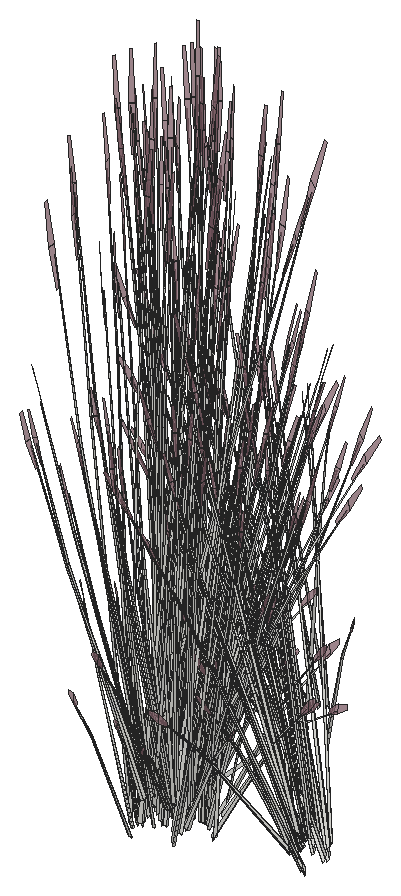
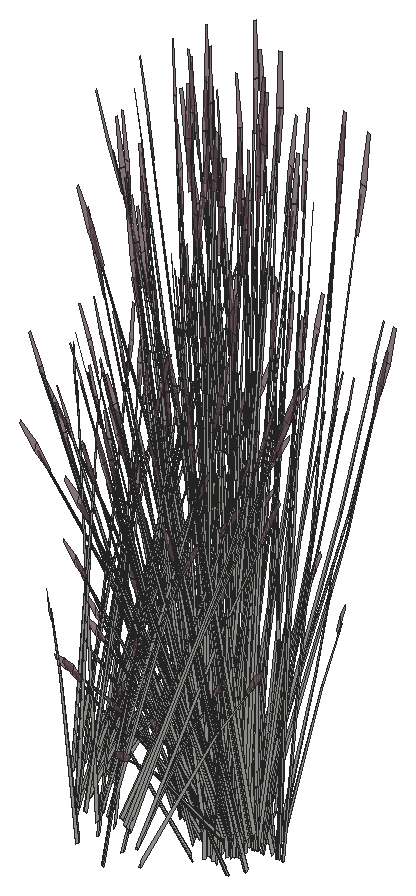
# SketchUp Ruby script. Lengths in inches.
U = 1.inch
M = Sketchup.active_model
def pt(a) = Geom::Point3d.new(a.map { |v| v * U })
def face(e, loops, mat)
  f = e.add_face(loops[0].map { |a| pt(a) })
  loops[1..].each { |l| e.add_face(l.map { |a| pt(a) }).erase! }
  f.material = f.back_material = mat if mat
  f
end
# faces: each face lists its corners as indices into pts; further lists are holes
def faces(e, pts, list, mat = nil) = list.each { |f| face(e, (f[0].is_a?(Array) ? f : [f]).map { |l| l.map { |i| pts[i] } }, mat) }
# xy, xz, yz: faces in a plane at the given z, y or x. An outline is a flat list of corners, or four numbers for a rectangle; further outlines are holes
def ring(l) = l.size == 4 ? [[l[0], l[1]], [l[2], l[1]], [l[2], l[3]], [l[0], l[3]]] : l.each_slice(2).to_a
def flat(e, list, mat, &to3) = list.each { |f| face(e, (f[0].is_a?(Array) ? f : [f]).map { |l| ring(l).map { |u, v| to3.(u, v) } }, mat) }
def xy(e, z, list, mat = nil) = flat(e, list, mat) { |x, y| [x, y, z] }
def xz(e, y, list, mat = nil) = flat(e, list, mat) { |x, z| [x, y, z] }
def yz(e, x, list, mat = nil) = flat(e, list, mat) { |y, z| [x, y, z] }
def lines(e, pts, list) = list.each { |a, b| e.add_line(pt(pts[a]), pt(pts[b])) }
# prism: a flat outline (further loops are holes) pulled along v
def prism(e, loops, v, mat = nil)
  f = face(e, loops, mat); d = Geom::Vector3d.new(v.map { |x| x * U })
  f.pushpull(f.normal.samedirection?(d) ? d.length : -d.length)
end
def box(e, o, s, mat = nil) = prism(e, [[o, [o[0] + s[0], o[1], o[2]], [o[0] + s[0], o[1] + s[1], o[2]], [o[0], o[1] + s[1], o[2]]]], [0, 0, s[2]], mat)
def at(x, y, z, deg = 0) = Geom::Transformation.translation(pt([x, y, z])) * Geom::Transformation.rotation(ORIGIN, Z_AXIS, deg.degrees)
def axes(o, x, y, z) = Geom::Transformation.new([*x, 0, *y, 0, *z, 0, *pt(o).to_a, 1])
def part(name) = M.definitions.add(name)
# library, detail: a bought-in or finely detailed component or shape, given as its bounding box
def library(name, o, s) = part(name).tap { |d| box(d.entities, o, s) }
def detail(e, o, s) = box(e.add_group.entities, o, s)
def put(e, d, t, mat = nil) = e.add_instance(d, t).tap { |i| i.material = mat if mat }
def group(e, t, mat = nil) = e.add_group.tap { |g| g.transformation = t; g.material = mat if mat }.entities
root = M.entities
M.materials.add("LightPink_Translucent").color = [144, 107, 117]
M.materials["LightPink_Translucent"].alpha = 0.75
c1 = part("blade")
p = [[2.15,0.21,22],[0,0.17,0],[0.09,0.45,0],[2.18,0.31,22],[2.29,0.31,22],[0.38,0.45,0],
  [2.48,0.24,33],[2.49,0.24,33],[2.48,0.22,33]]
faces(c1.entities,p,[[0,1,2,3],[4,5,2,3],[6,3,4,7],[8,0,3,6]])
c2 = part("seeds")
p = [[0.3,-0.1,1.38],[-0.01,-0.03,1.59],[-0.01,-0.03,0.03],[0.14,-0.07,-0.07],[0.29,-0.03,3],[0.15,0.01,3.11]]
faces(c2.entities,p,[[0,1,2,3],[1,0,4,5]],"LightPink_Translucent")
c3 = part("blade with seeds")
put(c3.entities,c1,at(0,0,0))
put(c3.entities,c2,axes([2.4,0.25,30.99],[1.5799,-0.05474,1.17369],[-0.12525,1.92788,0.29478],[-0.07173,-0.02425,1.56792]))
put(root,c3,axes([494.1,110.7,1.21],[-0.7111,0.30552,-0.49651],[-0.42504,-0.54784,0],[-0.16196,0.06958,1.57504]))
put(root,c3,axes([489.89,107.66,1.21],[0,-0.61104,-0.49651],[0.85008,0,0],[0,-0.13917,1.57504]))
put(root,c3,axes([490.25,108.22,1.67],[0,0.61104,0.49651],[-0.85008,0,0],[0,-0.13917,1.57504]))
put(root,c3,axes([494.14,110.54,1.39],[-0.46912,-0.61443,-0.05142],[0.79476,-0.34146,0.51607],[-0.19584,0.0585,1.6363]))
put(root,c3,axes([491.13,110.26,4.2],[0.54391,0.41056,-0.5672],[-0.57458,0.35956,-0.43934],[-0.08276,0.2086,1.08528]))
put(root,c3,axes([495.39,119.16,7.78],[-0.64788,-0.29534,-0.71045],[0.46044,-0.51755,0.08574],[-0.23473,-0.17635,1.00501]))
put(root,c3,axes([495.09,119.17,7.48],[-0.74975,0.14525,-0.51099],[-0.13115,-0.55007,-0.3958],[-0.20138,-0.15763,0.97773]))
put(root,c3,axes([493.93,110.46,1.22],[-0.70886,-0.15119,-0.30978],[0.17848,-0.53243,0.30978],[-0.1429,0.0614,1.38974]))
put(root,c3,axes([490.89,109.95,4.24],[0.5141,-0.32171,0.35414],[0.48666,0.36734,-0.4572],[-0.07405,0.18664,0.87481]))
put(root,c3,axes([492.11,108.36,1.86],[-0.85568,-0.29155,-0.29095],[0.41201,-0.61537,-0.50002],[-0.02689,-0.15109,1.59708]))
put(root,c3,axes([494.34,108.18,2.03],[-0.02076,-0.57531,1.41272],[0.93937,0.14913,0.59816],[-0.22217,0.31481,1.3335]))
put(root,c3,axes([494.125,118.67,4.29],[-0.0736,0.08049,1.76342],[-0.74378,0.17355,-0.26939],[-0.17968,-0.15788,0.30037]))
put(root,c3,axes([490.5625,110.04,4.59],[0.83505,0.03027,-0.13498],[-0.02282,0.57322,-0.74919],[-0.05801,0.22077,1.13838]))
put(root,c3,axes([490.54,110.875,2.02],[0.69024,-0.1082,0.06507],[0.15868,0.43593,-0.86304],[-0.04376,0.22067,0.7736]))
put(root,c3,axes([493.81,108.92,1.86],[0.08854,0.69723,-0.29095],[-0.92215,0.04216,-0.50002],[-0.16238,0.09287,1.59708]))
put(root,c3,axes([491.73,107.74,1.29],[-0.31203,-0.62659,-0.69835],[0.89884,-0.22566,-0.18329],[-0.03449,-0.21218,1.54149]))
put(root,c3,axes([493.77,105.75,4.23],[-0.74352,0.28449,-0.1216],[-0.36538,-0.50492,-0.67495],[-0.0981,-0.21277,1.02557]))
put(root,c3,axes([493.13,105.78,3.875],[-0.7469,-0.15318,-0.51099],[0.25601,-0.52518,-0.3958],[-0.06849,-0.21144,0.97773]))
put(root,c3,axes([491.75,109.67,3.07],[-0.0186,-0.23452,1.71376],[0.80601,0.15558,0.13857],[-0.04985,0.33422,0.73262]))
put(root,c3,axes([490.25,107.67,1.22],[0.53038,-0.38124,-0.30978],[0.53038,0.38124,0.30978],[0,-0.1228,1.38974]))
put(root,c3,axes([492.65,105.2,1.32],[-0.52505,0.35054,-0.03893],[-0.48109,-0.38392,-0.17649],[-0.03387,-0.10878,0.58215]))
put(root,c3,axes([492.43,108.66,1.55],[0.96033,0.12874,0.45755],[-0.19544,0.7271,0.17955],[-0.14034,-0.07021,1.58856]))
put(root,c3,axes([492.1875,108.53,1.91],[-0.36864,0.55059,0.44739],[-0.76598,-0.26498,-0.21531],[0,-0.12692,1.43643]))
put(root,c3,axes([493.4,105.88,4.17],[-0.36264,-0.49684,-0.71045],[0.74649,-0.27689,0.08574],[-0.0848,-0.24006,1.00501]))
put(root,c3,axes([494.67,118.35,5.39],[-0.04601,0.19989,1.43002],[-0.67263,0.16733,-0.30754],[-0.15723,-0.25836,0.61141]))
put(root,c3,axes([494.89,118.87,6.68],[0.17368,0.19618,1.71376],[-0.80256,0.16516,0.13857],[-0.18139,-0.30799,0.73262]))
put(root,c3,axes([491.92,109.82,1.67],[0.81646,-0.16218,0.17642],[0.20161,0.60355,0.35086],[-0.07282,-0.08794,1.60407]))
put(root,c3,axes([495.17,118.77,7.33],[-0.11735,-0.49217,-0.35414],[0.67083,-0.12996,0.4572],[-0.18018,-0.14104,0.87481]))
put(root,c3,axes([492.97,109.92,1.39],[-0.76598,-0.27433,0],[0.36864,-0.57001,0],[0,0,1.62707]))
put(root,c3,axes([493.54,105.95,4.24],[-0.22906,0.4699,0.35414],[-0.66828,-0.13705,-0.4572],[-0.06128,-0.18919,0.87481]))
put(root,c3,axes([494.74,110.61,1.57],[0.47504,0.61229,0],[-0.79476,0.34146,-0.51607],[-0.18101,0.07777,1.63711]))
put(root,c3,axes([492.32,110.87,4.26],[-0.74868,-0.15974,0.53283],[0.25601,-0.52518,0.43934],[0.04499,0.20653,1.10256]))
put(root,c3,axes([492.125,110.91,3.92],[-0.55987,0.20767,0.0643],[-0.27403,-0.37869,0.50621],[0.05407,0.16693,0.77189]))
put(root,c3,axes([494.35,109.86,1.67],[0.21949,-0.60727,0.17642],[0.8032,0.17185,0.35086],[-0.13875,0.00296,1.60407]))
put(root,c3,axes([493.98,109.05,1.81],[0.56134,0.36712,0.1448],[-0.46823,0.41419,-0.41347],[-0.13033,0.05599,1.26744]))
put(root,c3,axes([493.78,108.6,1.49],[-0.70674,-0.52593,-0.06131],[0.70717,-0.52625,0],[-0.02468,-0.01837,1.75571]))
put(root,c3,axes([493.96,108.78,1.91],[0.82508,-0.03772,0.44739],[0.07462,0.62614,-0.21531],[-0.14771,0.06346,1.43643]))
put(root,c3,axes([494.16,110.22,1.52],[0.95122,0.19861,0.30756],[-0.23797,0.7099,-0.36492],[-0.15744,0.08885,1.64885]))
put(root,c3,axes([494.4375,118.03,5.57],[0.39634,0.21267,1.1486],[-0.57721,0.12784,0.84392],[-0.1235,-0.16344,0.25299]))
put(root,c3,axes([492.78,104.78,0.6875],[-0.12744,0.02202,1.76342],[-0.70477,-0.24781,-0.26939],[0.01183,-0.2067,0.30037]))
put(root,c3,axes([494.57,110.18,1.67],[0.7111,-0.30552,0.49651],[0.42504,0.54784,0],[-0.16196,0.06958,1.57504]))
put(root,c3,axes([493.47,105.46,3.72],[0.22906,-0.4699,-0.35414],[0.66828,0.13705,0.4572],[-0.06128,-0.18919,0.87481]))
put(root,c3,axes([492.35,107.99,1.55],[0.33034,0.68327,0.45755],[-0.94388,0.2376,0.17955],[0.01154,-0.12555,1.58856]))
put(root,c3,axes([492.2,107.91,1.4],[0.36864,-0.55059,-0.44739],[0.76598,0.26498,0.21531],[0,-0.12692,1.43643]))
put(root,c3,axes([493.14,109.68,1.4],[-0.24791,-0.5268,0],[0.70791,-0.18448,0],[0,0,1.54371]))
put(root,c3,axes([492.24,110.79,0.6875],[0.12297,-0.03325,1.76342],[0.73967,0.18301,-0.26939],[0.02163,0.20626,0.30037]))
put(root,c3,axes([492.41,110.98,3.72],[-0.22906,0.4699,-0.35414],[-0.66828,-0.13705,0.4572],[0.06128,0.18919,0.87481]))
put(root,c3,axes([494.14,108.64,1.4],[-0.36864,0.55059,-0.44739],[-0.76598,-0.26498,0.21531],[0,0.12692,1.43643]))
put(root,c3,axes([493.75,105.52,3.92],[0.55987,-0.20767,0.0643],[0.27403,0.37869,0.50621],[-0.05407,-0.16693,0.77189]))
put(root,c3,axes([491.93,111.8125,3.91],[0.09631,0.0984,1.74944],[0.77725,0.03866,-0.27667],[0.07816,0.217,0.14031]))
put(root,c3,axes([495.6,108.31,1.67],[-0.59697,-0.44509,0.17642],[0.60159,-0.4317,0.35086],[-0.06593,0.0909,1.60407]))
put(root,c3,axes([493.54,108.05,1.4],[0,-0.70701,0],[0.95008,0,0],[0,0,1.79456]))
put(root,c3,axes([493.55,105.56,3.93],[0.74868,0.15974,0.48003],[-0.25601,0.52518,0.3958],[-0.04499,-0.20653,0.9933]))
put(root,c3,axes([492.66,108.18,1.625],[0.8561,0.29616,0.24065],[-0.41201,0.61537,0.50002],[0,-0.14185,1.60543]))
put(root,c3,axes([494.02,108.33,1.48],[0,0.70667,-0.05637],[-0.95008,0,0],[0,0.02221,1.79368]))
put(root,c3,axes([492.38,107.77,1.91],[-0.82508,0.03772,0.44739],[-0.07462,-0.62614,-0.21531],[0.14771,-0.06346,1.43643]))
put(root,c3,axes([492.33,110.48,4.24],[0.22906,-0.4699,0.35414],[0.66828,0.13705,-0.4572],[0.06128,0.18919,0.87481]))
put(root,c3,axes([492,106.69,1.67],[-0.21949,0.60727,0.17642],[-0.8032,-0.17185,0.35086],[0.13875,-0.00296,1.60407]))
put(root,c3,axes([493.5625,109.7,1.48],[0.33034,0.70197,-0.06012],[-0.94388,0.24598,0],[0.01154,0.02451,1.72173]))
put(root,c3,axes([491.6,105.94,1.57],[-0.47504,-0.61229,0],[0.79476,-0.34146,-0.51607],[0.18101,-0.07777,1.63711]))
put(root,c3,axes([492.48,110.56,4.17],[0.36264,0.49684,-0.71045],[-0.74649,0.27689,0.08574],[0.0848,0.24006,1.00501]))
put(root,c3,axes([496.29,108.78,1.39],[-0.94962,-0.00489,-0.04976],[0,-0.68292,0.49943],[-0.02984,0.15546,1.58352]))
put(root,c3,axes([495.35,120.88,4.9],[-0.31203,-0.62659,-0.69835],[0.89884,-0.22566,-0.18329],[-0.03449,-0.21218,1.54149]))
put(root,c3,axes([496.76,118.92,7.48],[-0.7469,-0.15318,-0.51099],[0.25601,-0.52518,-0.3958],[-0.06849,-0.21144,0.97773]))
put(root,c3,axes([494.43,106.72,1.67],[-0.81646,0.16218,0.17642],[-0.20161,-0.60355,0.35086],[0.07282,0.08794,1.60407]))
put(root,c3,axes([493.59,104.46,1.96],[0.09747,0.35631,1.1486],[-0.54071,-0.19735,0.84392],[0.05818,-0.18244,0.25299]))
put(root,c3,axes([493.23,112.16,4.84],[0.52505,-0.35054,-0.06488],[0.48109,0.38392,-0.29416],[0.03387,0.10878,0.97024]))
put(root,c3,axes([493.09,107.6,1.55],[-0.62999,0.55453,0.45755],[-0.74845,-0.4895,0.17955],[0.15188,-0.05534,1.58856]))
put(root,c3,axes([494.17,108.48,1.41],[0.53038,0.39469,0],[-0.53038,0.39469,0],[0,0,1.69266]))
put(root,c3,axes([494.16,108.02,1.91],[0.36864,-0.55059,0.44739],[0.76598,0.26498,-0.21531],[0,0.12692,1.43643]))
put(root,c3,axes([493.84,109.93,1.4],[0.76598,0.27433,0],[-0.36864,0.57001,0],[0,0,1.74954]))
put(root,c3,axes([492.75,110.66,3.875],[0.7469,0.15318,-0.51099],[-0.25601,0.52518,-0.3958],[0.06849,0.21144,0.97773]))
put(root,c3,axes([492.11,110.68,4.23],[0.74352,-0.28449,-0.1216],[0.36538,0.50492,-0.67495],[0.0981,0.21277,1.02557]))
put(root,c3,axes([493.91,107.89,1.57],[-0.96033,-0.12874,0.49198],[0.19544,-0.7271,0.19306],[0.14034,0.07021,1.70813]))
put(root,c3,axes([497.03,119.02,7.78],[-0.36264,-0.49684,-0.71045],[0.74649,-0.27689,0.08574],[-0.0848,-0.24006,1.00501]))
put(root,c3,axes([495.91,105.04,3.9],[-0.07716,0.04667,1.77383],[-0.75601,-0.15746,-0.16761],[-0.02737,-0.20368,0.31391]))
put(root,c3,axes([495.3125,106.39,4.23],[-0.83505,-0.03027,-0.1216],[0.02282,-0.57322,-0.67495],[0.05801,-0.22077,1.02557]))
put(root,c3,axes([496.09,108.88,1.22],[-0.53038,0.38124,-0.30978],[-0.53038,-0.38124,0.30978],[0,0.1228,1.38974]))
put(root,c3,axes([494.58,108.81,1.29],[0.2786,0.55945,-0.69212],[-0.80253,0.20149,-0.18165],[0.03079,0.18945,1.52773]))
put(root,c3,axes([494.18,108.21,1.4],[0.85008,0,0],[0,0.63259,0],[0,0,1.78407]))
put(root,c3,axes([494.99,106.48,4.24],[-0.5141,0.32171,0.35414],[-0.48666,-0.36734,-0.4572],[0.07405,-0.18664,0.87481]))
put(root,c3,axes([493.37,107.51,1.91],[-0.45644,-0.51287,0.44739],[0.69137,-0.36116,-0.21531],[0.14771,0.06346,1.43643]))
put(root,c3,axes([492.54,107.63,1.86],[-0.08854,-0.69723,-0.29095],[0.92215,-0.04216,-0.50002],[0.16238,-0.09287,1.59708]))
put(root,c3,axes([494.48,108.14,1.81],[0.70791,-0.1782,0.1448],[0.24791,0.50885,-0.41347],[0,0.11199,1.26744]))
put(root,c3,axes([494.74,106.18,3.875],[-0.54391,-0.41056,-0.51099],[0.57458,-0.35956,-0.3958],[0.08276,-0.2086,0.97773]))
put(root,c3,axes([494.24,108.18,1.86],[0.85568,0.29155,-0.29095],[-0.41201,0.61537,-0.50002],[0.02689,0.15109,1.59708]))
put(root,c3,axes([492.41,106.09,1.22],[0.70886,0.15119,-0.30978],[-0.17848,0.53243,0.30978],[0.1429,-0.0614,1.38974]))
put(root,c3,axes([494.39,105.45,1.78],[-0.21597,0.12368,1.43002],[-0.64681,-0.21647,-0.30754],[0.1199,-0.26922,0.61141]))
put(root,c3,axes([496.09,108.32,1.67],[0,-0.61104,0.49651],[0.85008,0,0],[0,0.13917,1.57504]))
put(root,c3,axes([496.46,108.89,1.21],[0,0.61104,-0.49651],[-0.85008,0,0],[0,0.13917,1.57504]))
put(root,c3,axes([496.4,117.91,4.29],[-0.12744,0.02202,1.76342],[-0.70477,-0.24781,-0.26939],[0.01183,-0.2067,0.30037]))
put(root,c3,axes([494.1875,110.74,3.93],[-0.75571,0.14023,0.48003],[-0.13115,-0.55007,0.3958],[0.17773,0.16212,0.9933]))
put(root,c3,axes([492.25,105.85,1.21],[0.7111,-0.30552,-0.49651],[0.42504,0.54784,0],[0.16196,-0.06958,1.57504]))
put(root,c3,axes([494.04,110.85,3.92],[-0.34533,0.38816,0.0643],[-0.49176,-0.22599,0.50621],[0.15898,0.12445,0.77189]))
put(root,c3,axes([493.17,109.57,3.07],[-0.17368,-0.19618,1.71376],[0.80256,-0.16516,0.13857],[0.18139,0.30799,0.73262]))
put(root,c3,axes([493.67,107.37,1.81],[0.14658,-0.54532,0.1448],[0.71613,0.09466,-0.41347],[0.13033,0.05599,1.26744]))
put(root,c3,axes([497.1,118.59,7.33],[0.22906,-0.4699,-0.35414],[0.66828,0.13705,0.4572],[-0.06128,-0.18919,0.87481]))
put(root,c3,axes([494.69,106.42,1.67],[-0.7111,-0.30552,0.49651],[0.42504,-0.54784,0],[0.16196,0.06958,1.57504]))
put(root,c3,axes([494.91,106.36,4.17],[0.01977,-0.56521,-0.71045],[0.83252,0.03796,0.08574],[0.08786,-0.23945,1.00501]))
put(root,c3,axes([494.07,109.61,1.38],[0.79769,-0.20732,-0.19198],[0.2803,0.59721,0.00008],[0.08805,-0.02292,1.73897]))
put(root,c3,axes([493.9375,110.41,4.24],[-0.11735,-0.49217,0.35414],[0.67083,-0.12996,-0.4572],[0.18018,0.14104,0.87481]))
put(root,c3,axes([494.09,107.83,1.4],[0.45644,0.51287,-0.44739],[-0.69137,0.36116,0.21531],[0.14771,0.06346,1.43643]))
put(root,c3,axes([494.39,107.57,3.67],[-0.65655,-0.31748,1.38283],[0.69326,-0.49431,0.59665],[0.21183,0.29789,1.33663]))
put(root,c3,axes([495.26,106.02,3.72],[0.5141,-0.32171,-0.35414],[0.48666,0.36734,0.4572],[0.07405,-0.18664,0.87481]))
put(root,c3,axes([493.28,111.09,3.9],[0.00225,-0.07398,1.77383],[0.65113,-0.32638,-0.16761],[0.22617,0.1165,0.31391]))
put(root,c3,axes([495.45,106.1875,3.92],[0.62439,0.02847,0.0643],[-0.01712,0.42991,0.50621],[0.06534,-0.16468,0.77189]))
put(root,c3,axes([495.38,110.16,1.96],[-0.4278,-0.1757,1.1486],[0.5524,-0.17852,0.84392],[0.14899,0.15122,0.25299]))
put(root,c3,axes([493.86,109.97,1.78],[0.01341,-0.20255,1.43002],[0.64074,-0.22625,-0.30754],[0.1978,0.24243,0.61141]))
put(root,c3,axes([496.07,105.48,3.91],[-0.00733,-0.12161,1.74944],[-0.61946,-0.35147,-0.27667],[0.09577,-0.21306,0.14031]))
put(root,c3,axes([493.09,107.1,1.25],[0.51177,-0.45928,-0.62353],[0.63575,0.41646,-0.16365],[0.20507,-0.11457,1.37633]))
put(root,c3,axes([495.25,106.15,3.93],[0.54105,0.41691,0.48003],[-0.57458,0.35956,0.3958],[0.0998,-0.1956,0.9933]))
put(root,c3,axes([495.34,106.69,1.22],[0.17848,0.53243,-0.30978],[-0.70886,0.15119,0.30978],[0.1429,0.0614,1.38974]))
put(root,c3,axes([496.67,108.43,1.57],[0.95008,0,0],[0,0.68292,-0.51607],[0,0.15554,1.63711]))
put(root,c3,axes([493.6,107.54,1.86],[0.76714,-0.40567,-0.29095],[0.51013,0.57321,-0.50002],[0.18927,0.05821,1.59708]))
put(root,c3,axes([495.45,110.96,1.86],[-0.48723,-0.01916,1.0506],[0.32177,-0.40701,0.58006],[0.19248,0.1446,0.8241]))
put(root,c3,axes([497.22,117.6,5.57],[0.09747,0.35631,1.1486],[-0.54071,-0.19735,0.84392],[0.05818,-0.18244,0.25299]))
put(root,c3,axes([495.88,107.47,4.24],[-0.66138,0.08733,0.35414],[-0.17464,-0.49921,-0.4572],[0.18953,-0.13408,0.87481]))
put(root,c3,axes([506.22,107.31,3.07],[0.31515,-0.01384,1.71376],[-0.20907,0.5998,0.13857],[-0.44912,-0.0371,0.73262]))
put(root,c3,axes([493.98,106.08,3.07],[-0.14147,0.21002,1.71376],[-0.59349,-0.43464,0.13857],[0.26773,-0.27089,0.73262]))
put(root,c3,axes([493.875,110.66,4.23],[0.45276,-0.52302,-0.1216],[0.65568,0.30132,-0.67495],[0.22792,0.14777,1.02557]))
put(root,c3,axes([491.66,107.18,0.79],[-0.74787,0.24464,1.28929],[-0.23804,-0.70192,0.50096],[0.45924,0.01168,1.46642]))
put(root,c3,axes([496.22,107.52,4.23],[-0.70283,-0.33692,-0.1216],[0.40491,-0.48793,-0.67495],[0.19857,-0.16961,1.02557]))
put(root,c3,axes([494.41,110.4,3.875],[0.74975,-0.14525,-0.51099],[0.13115,0.55007,-0.3958],[0.20138,0.15763,0.97773]))
put(root,c3,axes([498.37,119.3125,7.48],[-0.54391,-0.41056,-0.51099],[0.57458,-0.35956,-0.3958],[0.08276,-0.2086,0.97773]))
put(root,c3,axes([495.1,106.1,1.57],[0.47504,-0.61229,0],[0.79476,0.34146,-0.51607],[0.18101,0.07777,1.63711]))
put(root,c3,axes([495.9,105.83,0.6875],[-0.11372,-0.04814,1.76342],[-0.29211,-0.53779,-0.26939],[0.19706,-0.14594,0.30037]))
put(root,c3,axes([506.35,108.36,3.07],[0.26363,-0.12925,1.71376],[0.22195,0.59723,0.13857],[-0.41388,0.13498,0.73262]))
put(root,c3,axes([495.27,109.74,4.24],[-0.43232,-0.38257,0.35414],[0.49364,-0.36215,-0.4572],[0.25081,0.0551,0.87481]))
put(root,c3,axes([495.53,106.47,1.21],[0.7111,0.30552,-0.49651],[-0.42504,0.54784,0],[0.16196,0.06958,1.57504]))
put(root,c3,axes([505.53,109.38,1.78],[0.26405,0.05016,1.43002],[0.17019,0.51235,-0.30754],[-0.35868,0.0959,0.61141]))
put(root,c3,axes([495.67,110.09,3.92],[-0.03826,0.46465,0.0643],[-0.57772,-0.01274,0.50621],[0.2213,0.04862,0.77189]))
put(root,c3,axes([495.5,110.8125,0.6875],[0.05536,-0.08822,1.76342],[0.69692,-0.25981,-0.26939],[0.21129,0.13447,0.30037]))
put(root,c3,axes([495.72,109.94,3.93],[-0.56024,0.40262,0.48003],[-0.48318,-0.42758,0.3958],[0.26285,0.07427,0.9933]))
put(root,c3,axes([495.875,107.12,3.875],[-0.19519,-0.55794,-0.51099],[0.73919,-0.0976,-0.3958],[0.21183,-0.14986,0.97773]))
put(root,c3,axes([497.17,110,3.12],[-0.14542,-0.51365,-0.03492],[0.68734,-0.11809,-0.15832],[0.14353,0.03256,0.52218]))
put(root,c3,axes([495.98,108.67,4.24],[-0.63144,-0.17046,0.35414],[0.18417,-0.49731,-0.4572],[0.25423,-0.0456,0.87481]))
put(root,c3,axes([507.86,107.74,2.53],[0.21597,-0.08839,1.77064],[0.07448,0.61717,0.13857],[-0.4678,0.08189,0.63284]))
put(root,c3,axes([498.01,118.59,5.39],[-0.21597,0.12368,1.43002],[-0.64681,-0.21647,-0.30754],[0.1199,-0.26922,0.61141]))
put(root,c3,axes([494.5,107.64,1.25],[0.79037,0.10018,-0.62353],[-0.16679,0.61794,-0.16365],[0.23587,0.07488,1.37633]))
put(root,c3,axes([497.86,108,1.45],[-0.47106,-0.39072,-0.06488],[0.51591,-0.35801,-0.29416],[0.14618,-0.02521,0.97024]))
put(root,c3,axes([496.78,106.01,1.96],[-0.25308,0.31105,1.1486],[-0.21753,-0.4179,0.84392],[0.20902,-0.10472,0.25299]))
put(root,c3,axes([496.48,107.4,3.92],[0.52161,0.25698,0.0643],[-0.30368,0.36595,0.50621],[0.16723,-0.11831,0.77189]))
put(root,c3,axes([505.54,108.15,3.91],[-0.12407,0.07933,1.74944],[0.01055,0.57963,-0.27667],[-0.2844,0.07538,0.14031]))
put(root,c3,axes([507.16,106.75,4.17],[-0.75952,-0.01471,-0.71045],[0.05101,-0.61953,0.08574],[-0.32177,-0.06538,1.00501]))
put(root,c3,axes([498.54,119.5,7.78],[0.01977,-0.56521,-0.71045],[0.83252,0.03796,0.08574],[0.08786,-0.23945,1.00501]))
put(root,c3,axes([506.55,106.9,1.78],[0.14835,0.17012,1.43002],[-0.34183,0.46242,-0.30754],[-0.351,-0.11053,0.61141]))
put(root,c3,axes([496.33,107.29,3.93],[0.18844,0.56237,0.48003],[-0.73919,0.0976,0.3958],[0.21785,-0.13226,0.9933]))
put(root,c3,axes([505.9375,107.82,3.72],[-0.63144,-0.17046,-0.35414],[0.18417,-0.49731,0.4572],[-0.25423,0.0456,0.87481]))
put(root,c3,axes([506.8125,106.34,3.07],[0.28223,0.10528,1.71376],[-0.58406,0.44165,0.13857],[-0.36402,-0.19924,0.73262]))
put(root,c3,axes([494.33,108.96,3.07],[-0.28223,-0.10528,1.71376],[0.58406,-0.44165,0.13857],[0.36402,0.19924,0.73262]))
put(root,c3,axes([497.95,107.375,3.9],[-0.09924,-0.00464,1.77383],[-0.4121,-0.49725,-0.16761],[0.1655,-0.1635,0.31391]))
put(root,c3,axes([504.16,108.74,3.9],[0.09697,0.01639,1.77383],[0.29997,0.53988,-0.16761],[-0.1985,0.1417,0.31391]))
put(root,c3,axes([506.37,108.07,3.875],[-0.20584,0.55581,-0.51099],[-0.70573,-0.19051,-0.3958],[-0.28414,0.05097,0.97773]))
put(root,c3,axes([496.42,107.18,3.72],[0.66138,-0.08733,-0.35414],[0.17464,0.49921,0.4572],[0.18953,-0.13408,0.87481]))
put(root,c3,axes([495.89,107.35,4.17],[0.39688,-0.48213,-0.71045],[0.69548,0.34264,0.08574],[0.23697,-0.17468,1.00501]))
put(root,c3,axes([496.56,108.82,3.92],[0.27906,0.41663,0.0643],[-0.50888,0.20393,0.50621],[0.22432,-0.04024,0.77189]))
put(root,c3,axes([506.91,106.875,3.875],[-0.55171,0.40476,-0.51099],[-0.48318,-0.42758,-0.3958],[-0.28031,-0.06159,0.97773]))
put(root,c3,axes([495.89,109.94,3.72],[0.43232,0.38257,-0.35414],[-0.49364,0.36215,0.4572],[0.25081,0.0551,0.87481]))
put(root,c3,axes([506.02,108.04,0.6875],[0.01927,0.0963,1.76342],[-0.38846,0.5029,-0.26939],[-0.27592,-0.02535,0.30037]))
put(root,c3,axes([495.39,109.98,4.23],[0.04068,-0.62141,-0.1216],[0.77029,0.01698,-0.67495],[0.29667,0.04317,1.02557]))
put(root,c3,axes([496.25,108.84,4.23],[-0.38229,-0.5533,-0.1216],[0.6785,-0.2719,-0.67495],[0.28593,-0.073,1.02557]))
put(root,c3,axes([498.88,119.16,7.33],[0.5141,-0.32171,-0.35414],[0.48666,0.36734,0.4572],[0.07405,-0.18664,0.87481]))
put(root,c3,axes([496.5,108.67,3.93],[-0.21466,0.55714,0.48003],[-0.70573,-0.19051,0.3958],[0.27753,-0.03348,0.9933]))
put(root,c3,axes([506.13,105.74,3.9],[0.05633,0.06098,1.77383],[-0.27155,0.54815,-0.16761],[-0.27501,0.00397,0.31391]))
put(root,c3,axes([504.98,110.45,1.96],[0.31665,-0.27694,1.1486],[0.12495,0.43841,0.84392],[-0.22883,0.0785,0.25299]))
put(root,c3,axes([506.76,105.375,3.91],[-0.16348,-0.00431,1.74944],[-0.52047,0.43131,-0.27667],[-0.2777,-0.08813,0.14031]))
put(root,c3,axes([506.09,107.76,3.93],[0.21466,-0.55714,0.48003],[0.70573,0.19051,0.3958],[-0.27753,0.03348,0.9933]))
put(root,c3,axes([506.34,107.6,4.23],[0.38229,0.5533,-0.1216],[-0.6785,0.2719,-0.67495],[-0.28593,0.073,1.02557]))
put(root,c3,axes([507.2,106.45,4.23],[-0.04068,0.62141,-0.1216],[-0.77029,-0.01698,-0.67495],[-0.29667,-0.04317,1.02557]))
put(root,c3,axes([496.0625,109.61,3.91],[0.16299,-0.01033,1.74944],[0.44707,-0.47471,-0.27667],[0.28992,0.06266,0.14031]))
put(root,c3,axes([506.7,106.49,3.72],[-0.43232,-0.38257,-0.35414],[0.49364,-0.36215,0.4572],[-0.25081,-0.0551,0.87481]))
put(root,c3,axes([506.03,107.61,3.92],[-0.27906,-0.41663,0.0643],[0.50888,-0.20393,0.50621],[-0.22432,0.04024,0.77189]))
put(root,c3,axes([507.3125,108.76,3.07],[0.18977,-0.18775,1.71376],[0.47917,0.50677,0.13857],[-0.32866,0.23079,0.73262]))
put(root,c3,axes([506.17,109.26,3.72],[-0.66138,0.08733,-0.35414],[-0.17464,-0.49921,0.4572],[-0.18953,0.13408,0.87481]))
put(root,c3,axes([496.22,108.36,3.875],[0.20584,-0.55581,-0.51099],[0.70573,0.19051,-0.3958],[0.28414,-0.05097,0.97773]))
put(root,c3,axes([497.99,108.71,1.96],[-0.46945,0.10088,1.1486],[0.22097,-0.4169,0.84392],[0.24904,0.02853,0.25299]))
put(root,c3,axes([505.81,110.74,0.6875],[0.10192,0.06105,1.76342],[0.17281,0.56562,-0.26939],[-0.22588,0.12062,0.30037]))
put(root,c3,axes([505.66,107.41,1.96],[0.48508,-0.04372,1.1486],[-0.3077,0.38525,0.84392],[-0.23971,-0.05779,0.25299]))
put(root,c3,axes([496.47,106.9,1.78],[-0.27143,-0.0181,1.43002],[-0.27808,-0.48551,-0.30754],[0.33346,-0.13735,0.61141]))
put(root,c3,axes([497.6,119.22,6.68],[-0.14147,0.21002,1.71376],[-0.59349,-0.43464,0.13857],[0.26773,-0.27089,0.73262]))
put(root,c3,axes([496.65,108.61,3.72],[0.63144,0.17046,-0.35414],[-0.18417,0.49731,0.4572],[0.25423,-0.0456,0.87481]))
put(root,c3,axes([506.26,109.15,3.93],[-0.18844,-0.56237,0.48003],[0.73919,-0.0976,0.3958],[-0.21785,0.13226,0.9933]))
put(root,c3,axes([506.64,106.35,4.29],[0.62747,-0.45094,0.53763],[0.54116,0.47889,0.4433],[-0.29439,-0.08318,1.11249]))
put(root,c3,axes([495.43,109.6875,4.17],[0.75952,0.01471,-0.71045],[-0.05101,0.61953,0.08574],[0.32177,0.06538,1.00501]))
put(root,c3,axes([506.11,109.04,3.92],[-0.52161,-0.25698,0.0643],[0.30368,-0.36595,0.50621],[-0.16723,0.11831,0.77189]))
put(root,c3,axes([496.97,108.52,1.17],[-0.48937,0.07333,1.41583],[-0.07789,-0.58369,0.08104],[0.34275,-0.08835,0.80566]))
put(root,c3,axes([497.5,108.13,0.6875],[-0.03971,-0.09277,1.76342],[0.27541,-0.54264,-0.26939],[0.27782,-0.00781,0.30037]))
put(root,c3,axes([497.77,110.48,3.9],[-0.0687,-0.05349,1.77383],[0.15029,-0.57341,-0.16761],[0.27062,-0.03664,0.31391]))
put(root,c3,axes([507.17,109.23,3.07],[0.14147,-0.21002,1.71376],[0.59349,0.43464,0.13857],[-0.26773,0.27089,0.73262]))
put(root,c3,axes([494.93,108,3.07],[-0.31515,0.01384,1.71376],[0.20907,-0.5998,0.13857],[0.44912,0.0371,0.73262]))
put(root,c3,axes([499.52,118.97,4.29],[-0.11372,-0.04814,1.76342],[-0.29211,-0.53779,-0.26939],[0.19706,-0.14594,0.30037]))
put(root,c3,axes([506.6,107.77,4.24],[0.63144,0.17046,0.35414],[-0.18417,0.49731,-0.4572],[-0.25423,0.0456,0.87481]))
